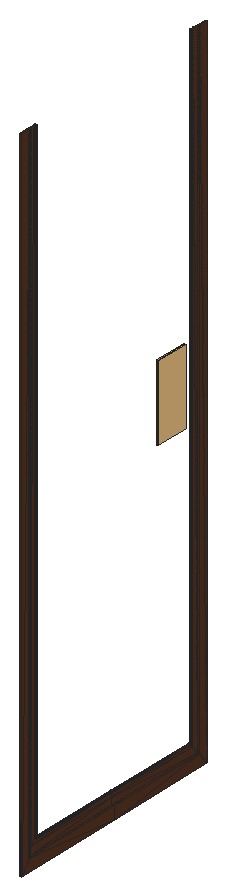
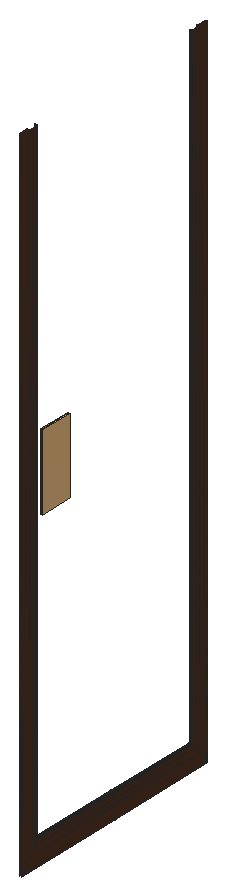
# SketchUp Ruby script. Lengths in inches.
U = 1.inch
M = Sketchup.active_model
def pt(a) = Geom::Point3d.new(a.map { |v| v * U })
def face(e, loops, mat)
  f = e.add_face(loops[0].map { |a| pt(a) })
  loops[1..].each { |l| e.add_face(l.map { |a| pt(a) }).erase! }
  f.material = f.back_material = mat if mat
  f
end
# faces: each face lists its corners as indices into pts; further lists are holes
def faces(e, pts, list, mat = nil) = list.each { |f| face(e, (f[0].is_a?(Array) ? f : [f]).map { |l| l.map { |i| pts[i] } }, mat) }
# xy, xz, yz: faces in a plane at the given z, y or x. An outline is a flat list of corners, or four numbers for a rectangle; further outlines are holes
def ring(l) = l.size == 4 ? [[l[0], l[1]], [l[2], l[1]], [l[2], l[3]], [l[0], l[3]]] : l.each_slice(2).to_a
def flat(e, list, mat, &to3) = list.each { |f| face(e, (f[0].is_a?(Array) ? f : [f]).map { |l| ring(l).map { |u, v| to3.(u, v) } }, mat) }
def xy(e, z, list, mat = nil) = flat(e, list, mat) { |x, y| [x, y, z] }
def xz(e, y, list, mat = nil) = flat(e, list, mat) { |x, z| [x, y, z] }
def yz(e, x, list, mat = nil) = flat(e, list, mat) { |y, z| [x, y, z] }
def lines(e, pts, list) = list.each { |a, b| e.add_line(pt(pts[a]), pt(pts[b])) }
# prism: a flat outline (further loops are holes) pulled along v
def prism(e, loops, v, mat = nil)
  f = face(e, loops, mat); d = Geom::Vector3d.new(v.map { |x| x * U })
  f.pushpull(f.normal.samedirection?(d) ? d.length : -d.length)
end
def box(e, o, s, mat = nil) = prism(e, [[o, [o[0] + s[0], o[1], o[2]], [o[0] + s[0], o[1] + s[1], o[2]], [o[0], o[1] + s[1], o[2]]]], [0, 0, s[2]], mat)
def at(x, y, z, deg = 0) = Geom::Transformation.translation(pt([x, y, z])) * Geom::Transformation.rotation(ORIGIN, Z_AXIS, deg.degrees)
def axes(o, x, y, z) = Geom::Transformation.new([*x, 0, *y, 0, *z, 0, *pt(o).to_a, 1])
def part(name) = M.definitions.add(name)
# library, detail: a bought-in or finely detailed component or shape, given as its bounding box
def library(name, o, s) = part(name).tap { |d| box(d.entities, o, s) }
def detail(e, o, s) = box(e.add_group.entities, o, s)
def put(e, d, t, mat = nil) = e.add_instance(d, t).tap { |i| i.material = mat if mat }
def group(e, t, mat = nil) = e.add_group.tap { |g| g.transformation = t; g.material = mat if mat }.entities
root = M.entities
M.materials.add("Material \#0").color = [86, 53, 35]
M.materials.add("Material \#1").color = [140, 140, 140]
c1 = part("3DGeom~19_Defintion")
xy(c1.entities,0,[[-6.28,-215.79,-994.45,-208.55,-13.52,-208.55],[-994.45,-215.79,-994.45,-208.55,-6.28,-215.79],[-6.28,-215.79,-13.52,-208.55,-13.52,0],[-6.28,-215.79,-13.52,0,-6.28,0],[-13.52,0,-13.52,208.55,-6.28,215.79],
  [-13.52,0,-6.28,215.79,-6.28,0],[-994.45,208.55,-6.28,215.79,-13.52,208.55],[-994.45,208.55,-994.45,215.79,-6.28,215.79]],"Material \#0")
p = [[-13.52,-208.55,0],[-994.45,-208.55,0],[-994.45,-207.81,0.07],[-14.25,-207.81,0.07],[-13.52,-208.55,0],[-14.25,-207.81,0.07],
  [-14.25,0,0.07],[-13.52,0,0],[-13.52,208.55,0],[-14.25,207.81,0.07],[-13.52,208.55,0],[-14.25,207.81,0.07],
  [-994.45,207.81,0.07],[-994.45,208.55,0],[-994.45,-207.21,0.27],[-994.45,-207.21,0.27],[-14.86,-207.21,0.27],[-14.86,-207.21,0.27],
  [-14.86,0,0.27],[-14.86,0,0.27],[-14.86,0,0.27],[-14.86,0,0.27],[-14.86,207.21,0.27],[-14.86,207.21,0.27],
  [-994.45,207.21,0.27],[-994.45,207.21,0.27],[-14.86,-207.21,0.27],[-994.45,-207.21,0.27],[-994.45,-206.74,0.6],[-15.33,-206.74,0.6],
  [-14.86,-207.21,0.27],[-15.33,-206.74,0.6],[-15.33,0,0.6],[-14.86,0,0.27],[-14.86,207.21,0.27],[-15.33,206.74,0.6],
  [-14.86,207.21,0.27],[-15.33,206.74,0.6],[-994.45,206.74,0.6],[-994.45,207.21,0.27],[-994.45,-206.4,1.07],[-15.66,-206.4,1.07],
  [-15.66,-206.4,1.07],[-15.66,0,1.07],[-15.66,206.4,1.07],[-15.66,206.4,1.07],[-994.45,206.4,1.07],[-994.45,-206.2,1.68],
  [-15.86,-206.2,1.68],[-15.86,-206.2,1.68],[-15.86,0,1.68],[-15.86,206.2,1.68],[-15.86,206.2,1.68],[-994.45,206.2,1.68],
  [-994.45,-206.13,2.41],[-15.93,-206.13,2.41],[-15.93,-206.13,2.41],[-15.93,0,2.41],[-15.93,206.13,2.41],[-15.93,206.13,2.41],
  [-994.45,206.13,2.41],[-994.45,-206.13,71.16],[-994.45,-206.22,71.59],[-15.79,-206.28,71.53],[-15.79,-206.28,71.53],[-15.84,0,71.59],
  [-15.93,0,71.16],[-15.79,206.28,71.53],[-15.79,206.28,71.53],[-994.45,206.22,71.59],[-994.45,206.13,71.16],[-15.79,-206.28,71.53],
  [-994.45,-206.48,71.84],[-994.45,-206.9,71.93],[-15.16,-206.9,71.93],[-15.79,-206.28,71.53],[-15.79,-206.28,71.53],[-15.16,-206.9,71.93],
  [-15.16,0,71.93],[-994.45,-206.48,71.84],[-15.59,0,71.84],[-15.79,-206.28,71.53],[-15.59,0,71.84],[-15.79,206.28,71.53],
  [-15.16,206.9,71.93],[-15.59,0,71.84],[-15.79,206.28,71.53],[-994.45,206.48,71.84],[-15.79,206.28,71.53],[-15.16,206.9,71.93],
  [-994.45,206.9,71.93],[-994.45,206.48,71.84],[-15.79,206.28,71.53],[-994.45,-227.27,72.01],[5.41,-227.47,72.33],[4.78,-226.84,71.93],
  [4.78,-226.84,71.93],[5.41,-227.47,72.33],[5.21,0,72.01],[-994.45,-226.84,71.93],[-994.45,-227.27,72.01],[5.21,0,72.01],
  [4.78,0,71.93],[4.78,226.84,71.93],[5.21,0,72.01],[5.21,0,72.01],[5.41,227.47,72.33],[4.78,226.84,71.93],
  [5.41,227.47,72.33],[-994.45,227.27,72.01],[-994.45,227.27,72.01],[-994.45,226.84,71.93],[-994.45,-227.27,72.01],[-994.45,-227.53,72.27],
  [5.41,-227.47,72.33],[5.41,-227.47,72.33],[5.47,0,72.27],[5.21,0,72.01],[5.41,227.47,72.33],[5.41,227.47,72.33],
  [-994.45,227.53,72.27],[-994.45,227.27,72.01],[-994.45,-227.61,72.7],[-994.45,-227.61,74.4375],[-994.45,-227.61,74.4375],[5.55,-227.61,74.4375],
  [5.55,-227.61,74.4375],[5.55,0,74.4375],[5.55,0,72.7],[5.55,227.61,74.4375],[5.55,227.61,74.4375],[-994.45,227.61,74.4375],
  [-994.45,227.61,74.4375],[-994.45,227.61,72.7]]
faces(c1.entities,p,[[0,1,2],[2,3,0],[4,5,6],[6,7,4],[8,7,6],[6,9,8],[10,11,12],[12,13,10],
  [3,2,14],[15,16,3],[5,17,18],[19,6,5],[9,6,20],[21,22,9],[11,23,24],[25,12,11],
  [26,27,28],[28,29,26],[30,31,32],[32,33,30],[34,33,32],[32,35,34],[36,37,38],[38,39,36],
  [29,28,40],[40,41,29],[31,42,43],[43,32,31],[35,32,43],[43,44,35],[37,45,46],[46,38,37],
  [41,40,47],[47,48,41],[42,49,50],[50,43,42],[44,43,50],[50,51,44],[45,52,53],[53,46,45],
  [48,47,54],[54,55,48],[49,56,57],[57,50,49],[51,50,57],[57,58,51],[52,59,60],[60,53,52],
  [61,62,63],[64,65,66],[66,65,67],[68,69,70],[71,72,73],[73,74,75],[76,77,78],[62,79,63],
  [78,80,76],[81,82,65],[83,80,78],[78,84,83],[65,85,86],[68,87,69],[88,89,90],[90,91,92],
  [93,94,95],[96,97,98],[95,99,100],[101,102,96],[103,102,104],[105,106,103],[107,108,109],[110,111,107],
  [112,113,114],[115,116,117],[117,116,118],[119,120,121],[114,122,123],[124,125,114],[113,122,114],[115,126,127],
  [127,128,115],[115,128,116],[118,128,127],[127,129,118],[116,128,118],[119,130,131],[132,133,119],[119,133,120]],"Material \#0")
c2 = part("3DGeom~21_Defintion")
xy(c2.entities,73.08,[[-976.3,-241.71,23.7,-241.71,-976.3,-223.46],[23.7,-241.71,5.45,-223.46,-976.3,-223.46],[23.7,-241.71,23.7,0,5.45,-223.46],[5.45,-223.46,23.7,0,5.45,0],[23.7,0,23.7,241.71,5.45,223.46],
  [5.45,0,23.7,0,5.45,223.46],[-976.3,223.46,23.7,241.71,-976.3,241.71],[-976.3,223.46,5.45,223.46,23.7,241.71]],"Material \#0")
c3 = part("3DGeom~22_Defintion")
xz(c3.entities,-210.625,[[-1016.13,2.47,-1016.13,9.96,-16.28,2.47],[-16.28,2.47,-1016.13,9.96,-16.28,9.96],[-1016.13,9.96,-1016.13,51.7,-16.28,51.7],[-1016.13,9.96,-16.28,51.7,-16.28,9.96],[-1016.13,51.7,-1016.13,72.71,-16.28,51.7]],"Material \#0")
xz(c3.entities,210.625,[[-1016.13,2.47,-16.28,2.47,-1016.13,9.96],[-16.28,2.47,-16.28,9.96,-1016.13,9.96],[-1016.13,9.96,-16.28,51.7,-1016.13,51.7],[-1016.13,9.96,-16.28,9.96,-16.28,51.7],[-1016.13,51.7,-16.28,51.7,-1016.13,72.71]],"Material \#0")
yz(c3.entities,-16.28,[[-210.625,2.47,-210.625,9.96,0,9.96],[-210.625,2.47,0,9.96,0,2.47],[0,2.47,0,9.96,210.625,2.47],[210.625,2.47,0,9.96,210.625,9.96],[-210.625,9.96,-210.625,51.7,0,51.7],
  [-210.625,9.96,0,51.7,0,9.96],[0,9.96,0,51.7,210.625,9.96],[210.625,9.96,0,51.7,210.625,51.7],[-210.625,51.7,0,72.71,0,51.7],[0,51.7,0,72.71,210.625,51.7]],"Material \#0")
p = [[-1016.13,-210.625,72.71],[-16.13,-210.77,73.09],[-16.28,-210.625,51.7],[-16.28,-210.625,51.7],[-16.13,-210.77,73.09],[-16.28,0,72.71],
  [-16.13,210.77,73.09],[-16.28,210.625,51.7],[-16.28,210.625,51.7],[-16.13,210.77,73.09],[-1016.13,210.625,72.71]]
faces(c3.entities,p,[[0,1,2],[3,4,5],[5,6,7],[8,9,10]],"Material \#0")
c4 = part("3DGeom~20_Defintion")
xy(c4.entities,0,[[-976.3,-241.71,-976.3,-223.46,23.7,-241.71],[23.7,-241.71,-976.3,-223.46,5.45,-223.46],[23.7,-241.71,5.45,-223.46,5.45,0],[23.7,-241.71,5.45,0,23.7,0],[-976.3,-223.46,-976.3,-211.85,5.45,-223.46],
  [5.45,-223.46,-976.3,-211.85,-6.16,-211.85],[5.45,-223.46,-6.16,-211.85,-6.16,0],[5.45,-223.46,-6.16,0,5.45,0],[-6.16,0,-6.16,211.85,5.45,223.46],[-6.16,0,5.45,223.46,5.45,0],
  [5.45,0,23.7,241.71,23.7,0],[5.45,0,5.45,223.46,23.7,241.71],[-976.3,211.85,-976.3,223.46,5.45,223.46],[-976.3,211.85,5.45,223.46,-6.16,211.85],[-976.3,223.46,-976.3,241.71,23.7,241.71],
  [-976.3,223.46,23.7,241.71,5.45,223.46]],"Material \#0")
c5 = part("3DGeom~18_Defintion")
xz(c5.entities,-241.71,[[-976.3,0,23.7,0,23.7,7.58],[-976.3,0,23.7,7.58,-976.3,7.58]],"Material \#0")
xz(c5.entities,241.71,[[-976.3,0,-976.3,7.58,23.7,7.58],[-976.3,0,23.7,7.58,23.7,0]],"Material \#0")
yz(c5.entities,23.7,[[-241.71,0,0,0,-241.71,7.58],[0,0,0,7.58,-241.71,7.58],[0,0,241.71,0,241.71,7.58],[0,0,241.71,7.58,0,7.58]],"Material \#0")
c6 = library("3DGeom~3_Defintion",[-83.33,-500,-350],[620.1,1000,533.33])
yz(root,155.64,[[443.39,50.76,443.4,50.76,443.39,60.79],[443.4,50.76,443.4,52.92,443.39,60.79],[443.4,52.92,443.4,60.79,443.39,60.79]],"Material \#1")
yz(root,155.78,[[443.39,50.76,443.39,60.79,443.4,50.76],[443.4,50.76,443.39,60.79,443.4,52.92],[443.4,52.92,443.39,60.79,443.4,60.79]],"Material \#1")
put(root,c1,axes([155.34,430.68,2.53],[0,0,-0.10404],[0,-0.07468,0],[0.00522,0,0]),"Material \#0")
put(root,c2,axes([155.34,430.68,2.53],[0,0,-0.10598],[0,-0.07607,0],[0.00532,0,0]),"Material \#0")
put(root,c3,axes([155.34,430.68,2.53],[0,0,-0.10182],[0,-0.07309,0],[0.00511,0,0]),"Material \#0")
put(root,c4,axes([155.34,430.68,2.53],[0,0,-0.10598],[0,-0.07607,0],[0.00532,0,0]),"Material \#0")
put(root,c5,axes([155.34,430.68,2.53],[0,0,-0.10598],[0,-0.07607,0],[0.00532,0,0]),"Material \#0")
put(root,c6,axes([155.66,444.02,55.77],[0,-0.00865,0],[0,0,-0.01205],[-0.00061,0,0]),"Material \#1")
